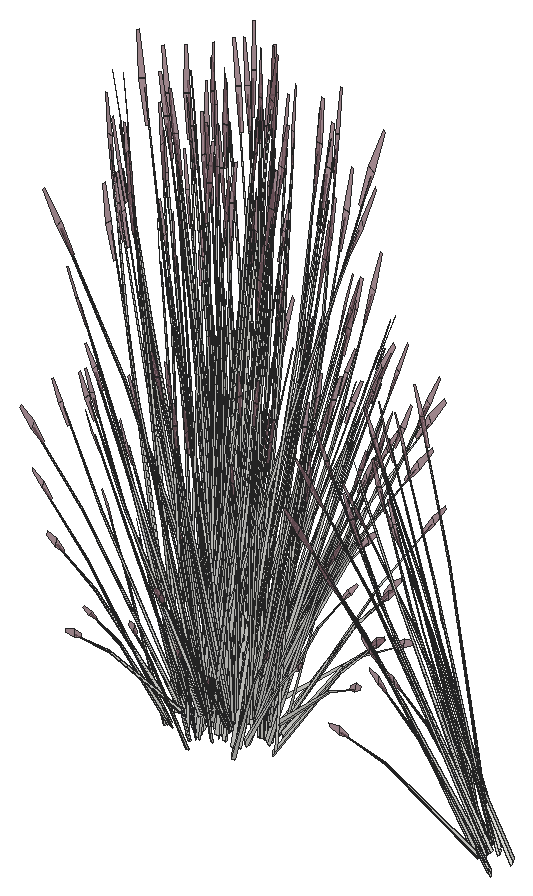
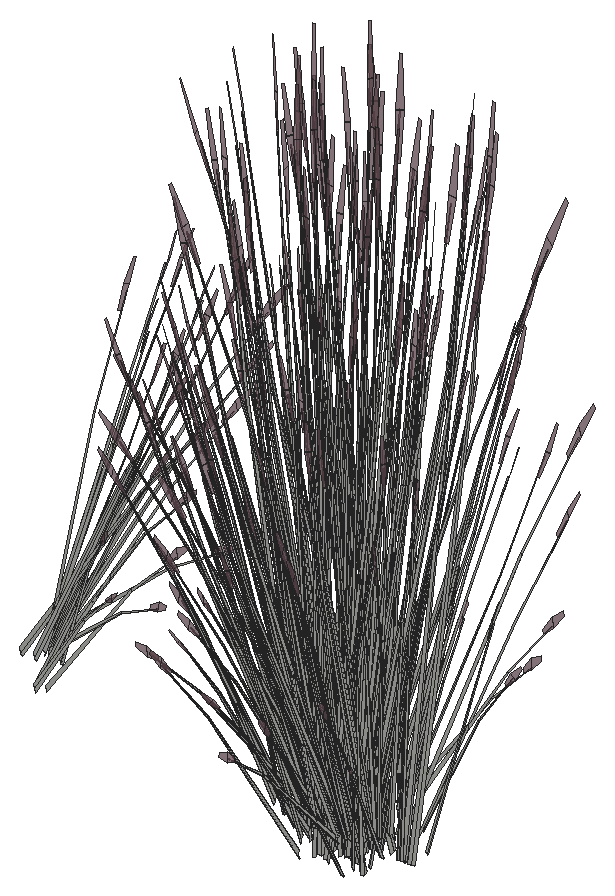
# SketchUp Ruby script. Lengths in inches.
U = 1.inch
M = Sketchup.active_model
def pt(a) = Geom::Point3d.new(a.map { |v| v * U })
def face(e, loops, mat)
  f = e.add_face(loops[0].map { |a| pt(a) })
  loops[1..].each { |l| e.add_face(l.map { |a| pt(a) }).erase! }
  f.material = f.back_material = mat if mat
  f
end
# faces: each face lists its corners as indices into pts; further lists are holes
def faces(e, pts, list, mat = nil) = list.each { |f| face(e, (f[0].is_a?(Array) ? f : [f]).map { |l| l.map { |i| pts[i] } }, mat) }
# xy, xz, yz: faces in a plane at the given z, y or x. An outline is a flat list of corners, or four numbers for a rectangle; further outlines are holes
def ring(l) = l.size == 4 ? [[l[0], l[1]], [l[2], l[1]], [l[2], l[3]], [l[0], l[3]]] : l.each_slice(2).to_a
def flat(e, list, mat, &to3) = list.each { |f| face(e, (f[0].is_a?(Array) ? f : [f]).map { |l| ring(l).map { |u, v| to3.(u, v) } }, mat) }
def xy(e, z, list, mat = nil) = flat(e, list, mat) { |x, y| [x, y, z] }
def xz(e, y, list, mat = nil) = flat(e, list, mat) { |x, z| [x, y, z] }
def yz(e, x, list, mat = nil) = flat(e, list, mat) { |y, z| [x, y, z] }
def lines(e, pts, list) = list.each { |a, b| e.add_line(pt(pts[a]), pt(pts[b])) }
# prism: a flat outline (further loops are holes) pulled along v
def prism(e, loops, v, mat = nil)
  f = face(e, loops, mat); d = Geom::Vector3d.new(v.map { |x| x * U })
  f.pushpull(f.normal.samedirection?(d) ? d.length : -d.length)
end
def box(e, o, s, mat = nil) = prism(e, [[o, [o[0] + s[0], o[1], o[2]], [o[0] + s[0], o[1] + s[1], o[2]], [o[0], o[1] + s[1], o[2]]]], [0, 0, s[2]], mat)
def at(x, y, z, deg = 0) = Geom::Transformation.translation(pt([x, y, z])) * Geom::Transformation.rotation(ORIGIN, Z_AXIS, deg.degrees)
def axes(o, x, y, z) = Geom::Transformation.new([*x, 0, *y, 0, *z, 0, *pt(o).to_a, 1])
def part(name) = M.definitions.add(name)
# library, detail: a bought-in or finely detailed component or shape, given as its bounding box
def library(name, o, s) = part(name).tap { |d| box(d.entities, o, s) }
def detail(e, o, s) = box(e.add_group.entities, o, s)
def put(e, d, t, mat = nil) = e.add_instance(d, t).tap { |i| i.material = mat if mat }
def group(e, t, mat = nil) = e.add_group.tap { |g| g.transformation = t; g.material = mat if mat }.entities
root = M.entities
M.materials.add("LightPink_Translucent").color = [144, 107, 117]
M.materials["LightPink_Translucent"].alpha = 0.75
c1 = part("blade")
p = [[2.15,0.21,22],[0,0.17,0],[0.09,0.45,0],[2.18,0.31,22],[2.29,0.31,22],[0.38,0.45,0],
  [2.48,0.24,33],[2.49,0.24,33],[2.48,0.22,33]]
faces(c1.entities,p,[[0,1,2,3],[4,5,2,3],[6,3,4,7],[8,0,3,6]])
c2 = part("seeds")
p = [[0.3,-0.1,1.38],[-0.01,-0.03,1.59],[-0.01,-0.03,0.03],[0.14,-0.07,-0.07],[0.29,-0.03,3],[0.15,0.01,3.11]]
faces(c2.entities,p,[[0,1,2,3],[1,0,4,5]],"LightPink_Translucent")
c3 = part("blade with seeds")
put(c3.entities,c1,at(0,0,0))
put(c3.entities,c2,axes([2.4,0.25,30.99],[1.5799,-0.05474,1.17369],[-0.12525,1.92788,0.29478],[-0.07173,-0.02425,1.56792]))
put(root,c3,axes([821.01,272.59,2.53],[0.40003,-0.04673,0.17707],[0.10563,0.26712,-0.2286],[-0.11464,0.07175,0.4374]))
put(root,c3,axes([821.24,273.87,1.3],[0.14502,-0.05158,0.71501],[0.35805,0.15552,-0.15377],[-0.10657,0.13457,0.3057]))
put(root,c3,axes([821.03,270.93,1.0625],[-0.13257,0.26698,-0.01946],[-0.40802,-0.08212,-0.08825],[-0.06195,-0.04367,0.29107]))
put(root,c3,axes([822.09,270.02,2.35],[-0.00857,0.03919,0.88692],[-0.42284,0.14223,-0.08381],[-0.12443,-0.0727,0.15695]))
put(root,c3,axes([821.64,270.59,1.3],[-0.02783,0.10696,0.71501],[-0.40683,0.08954,-0.15377],[-0.0951,-0.13825,0.3057]))
put(root,c3,axes([821.77,270.87,1.9375],[0.10505,0.10498,0.85688],[-0.48542,0.08838,0.06928],[-0.10971,-0.1648,0.36631]))
put(root,c3,axes([822.67,272.62,1.33],[-0.46399,0.21707,-0.14548],[-0.30855,-0.30672,-0.25001],[-0.11448,-0.03115,0.79854]))
put(root,c3,axes([821.38,273.3,2.37],[-0.32725,-0.22308,0.24001],[0.34753,-0.1924,0.1979],[-0.06036,0.10466,0.49665]))
put(root,c3,axes([821.94,270.8125,2.26],[-0.07098,-0.26335,-0.17707],[0.40574,-0.06954,0.2286],[-0.10898,-0.07547,0.4374]))
put(root,c3,axes([820.81,272.14,1.1875],[-0.57465,0,0],[0,-0.36542,-0.25804],[0,-0.08323,0.81856]))
put(root,c3,axes([821.62,273.07,1.01],[-0.10795,-0.28489,-0.15489],[0.42874,-0.0809,0.15489],[-0.08643,-0.03285,0.69487]))
put(root,c3,axes([821.26,273.28,2.37],[-0.37765,-0.01523,0.03215],[0.01035,-0.23004,0.2531],[-0.03952,0.08812,0.38595]))
put(root,c3,axes([821.38,273.37,2.26],[-0.31095,0.17214,-0.17707],[-0.29435,-0.19656,0.2286],[-0.04479,0.09987,0.4374]))
put(root,c3,axes([822.98,272.86,1.03],[-0.30954,0.24575,-0.31177],[-0.38452,-0.22284,-0.08182],[-0.12404,0.0613,0.68817]))
put(root,c3,axes([822.18,271.03,2.53],[0.07098,0.26335,0.17707],[-0.40574,0.06954,-0.2286],[-0.10898,-0.07547,0.4374]))
put(root,c3,axes([820.28,273.98,2.35],[0.05214,-0.01974,0.88692],[0.43092,0.1313,-0.08381],[-0.01013,0.10932,0.15695]))
put(root,c3,axes([821.26,272.05,1.17],[-0.42746,0.27488,0.15378],[-0.42772,-0.27199,-0.18246],[-0.01493,-0.07806,0.82443]))
put(root,c3,axes([823.01,272.81,1.66],[0.39713,0.13184,0.7563],[-0.38905,0.28403,0.29908],[-0.17427,-0.16834,0.63403]))
put(root,c3,axes([821.5,270.42,1.38],[0.23972,0.1138,0.5743],[-0.34912,0.06841,0.42196],[-0.0747,-0.08746,0.12649]))
put(root,c3,axes([823.1875,272.72,1.23],[-0.44875,-0.26316,-0.12596],[0.3776,-0.2955,0.27565],[-0.12084,0.03078,0.84108]))
put(root,c3,axes([822.37,272.46,1.11],[-0.27607,-0.27443,-0.2237],[0.41817,-0.19325,0.10766],[-0.08934,-0.03396,0.71822]))
put(root,c3,axes([821.59,273.1875,2.67],[-0.01196,0.30243,-0.3943],[-0.50354,-0.02031,0.04758],[-0.05314,0.12813,0.55778]))
put(root,c3,axes([821.58,274.04,1.38],[-0.01189,-0.19441,0.5743],[0.29719,0.13866,0.42196],[-0.05845,0.09266,0.12649]))
put(root,c3,axes([822,270.72,2.55],[0.51193,-0.08404,0.26881],[0.08885,0.32966,0.22165],[-0.1204,-0.09716,0.55625]))
put(root,c3,axes([822.96,272.66,1.11],[-0.49904,0.02018,-0.2237],[-0.04513,-0.33504,0.10766],[-0.08934,0.03396,0.71822]))
put(root,c3,axes([822.12,270.79,2.37],[0.20887,-0.2077,0.03215],[0.29744,0.12092,0.2531],[-0.09616,-0.06659,0.38595]))
put(root,c3,axes([822.01,273.22,1.24],[0.4301,0.16348,0.24825],[-0.25708,0.29314,0],[-0.09796,-0.03723,0.78752]))
put(root,c3,axes([821.42,273.61,1.68],[0.0101,-0.16879,0.77173],[0.45413,0.08915,0.10664],[-0.03935,0.17989,0.36441]))
put(root,c3,axes([822.41,272.62,1.22],[0.1218,-0.38743,-0.11714],[0.57753,0.06753,0.25635],[-0.10091,-0.0535,0.7822]))
put(root,c3,axes([822.62,272.71,1.31],[-0.08866,0.29179,0.0724],[-0.43315,-0.05065,-0.20674],[-0.07883,-0.02996,0.63372]))
put(root,c3,axes([822.57,270.17,2.36],[-0.07029,-0.04584,0.87472],[-0.46908,0.02906,-0.13834],[-0.07486,-0.10965,0.07015]))
put(root,c3,axes([823.48,273.53,1.01],[-0.4301,0.16348,-0.24825],[-0.25708,-0.29314,0],[-0.09796,0.03723,0.78752]))
put(root,c3,axes([820.9375,271.9,1.01],[0,-0.32696,-0.24825],[0.51416,0,0],[0,-0.07447,0.78752]))
put(root,c3,axes([821.16,272.2,1.24],[0,0.32696,0.24825],[-0.51416,0,0],[0,-0.07447,0.78752]))
put(root,c3,axes([823.51,273.4375,1.1],[-0.28374,-0.32877,-0.02571],[0.4807,-0.18271,0.25804],[-0.11845,0.0313,0.81815]))
put(root,c3,axes([821.69,273.29,2.5],[0.32898,0.21969,-0.2836],[-0.34753,0.1924,-0.21967],[-0.05006,0.11162,0.54264]))
put(root,c3,axes([823.38,273.4,1.01],[-0.42874,-0.0809,-0.15489],[0.10795,-0.28489,0.15489],[-0.08643,0.03285,0.69487]))
put(root,c3,axes([821.55,273.125,2.53],[0.31095,-0.17214,0.17707],[0.29435,0.19656,-0.2286],[-0.04479,0.09987,0.4374]))
put(root,c3,axes([822.28,272.28,1.33],[-0.51755,-0.15601,-0.14548],[0.2492,-0.32927,-0.25001],[-0.01626,-0.08084,0.79854]))
put(root,c3,axes([823.63,272.18,1.42],[-0.01255,-0.30784,0.70636],[0.56816,0.0798,0.29908],[-0.13438,0.16845,0.66675]))
put(root,c3,axes([821.35,273.17,2.7],[0.50507,0.0162,-0.06749],[-0.01381,0.30672,-0.3746],[-0.03508,0.11813,0.56919]))
put(root,c3,axes([821.34,273.62,1.41],[0.41748,-0.0579,0.03254],[0.09598,0.23326,-0.43152],[-0.02647,0.11808,0.3868]))
put(root,c3,axes([823.3125,272.57,1.33],[0.05355,0.37308,-0.14548],[-0.55775,0.02256,-0.25001],[-0.09822,0.04969,0.79854]))
put(root,c3,axes([822.05,271.94,1.05],[-0.18873,-0.33528,-0.34918],[0.54365,-0.12075,-0.09164],[-0.02086,-0.11353,0.77075]))
put(root,c3,axes([823.29,270.88,2.52],[-0.44971,0.15222,-0.0608],[-0.221,-0.27017,-0.33747],[-0.05933,-0.11385,0.51278]))
put(root,c3,axes([822.9,270.89,2.34],[-0.45175,-0.08196,-0.25549],[0.15485,-0.28101,-0.1979],[-0.04142,-0.11314,0.48886]))
put(root,c3,axes([822.07,272.97,1.9375],[-0.01125,-0.12549,0.85688],[0.48751,0.08325,0.06928],[-0.03015,0.17883,0.36631]))
put(root,c3,axes([821.16,271.9,1.01],[0.32079,-0.20399,-0.15489],[0.32079,0.20399,0.15489],[0,-0.06571,0.69487]))
put(root,c3,axes([822.61,270.58,1.0625],[-0.31757,0.18757,-0.01946],[-0.29098,-0.20543,-0.08825],[-0.02049,-0.05821,0.29107]))
put(root,c3,axes([822.48,272.43,1.18],[0.58084,0.06889,0.22877],[-0.11821,0.38906,0.08977],[-0.08488,-0.03757,0.79428]))
put(root,c3,axes([822.33,272.36,1.36],[-0.22297,0.29461,0.2237],[-0.4633,-0.14179,-0.10766],[0,-0.06791,0.71822]))
put(root,c3,axes([823.07,270.95,2.49],[-0.21934,-0.26585,-0.35523],[0.45151,-0.14816,0.04287],[-0.05129,-0.12845,0.5025]))
put(root,c3,axes([822.17,273.06,1.24],[0.49383,-0.08678,0.08821],[0.12194,0.32295,0.17543],[-0.04404,-0.04705,0.80203]))
put(root,c3,axes([822.8,273.11,1.1],[-0.4633,-0.14679,0],[0.22297,-0.30501,0],[0,0,0.81353]))
put(root,c3,axes([823.15,270.98,2.53],[-0.13855,0.25143,0.17707],[-0.4042,-0.07334,-0.2286],[-0.03706,-0.10123,0.4374]))
put(root,c3,axes([823.875,273.48,1.1875],[0.28732,0.32763,0],[-0.4807,0.18271,-0.25804],[-0.10948,0.04161,0.81856]))
put(root,c3,axes([822.41,273.62,2.53],[-0.45283,-0.08548,0.26641],[0.15485,-0.28101,0.21967],[0.02721,0.11051,0.55128]))
put(root,c3,axes([822.29,273.64,2.37],[-0.33863,0.11112,0.03215],[-0.16575,-0.20263,0.2531],[0.0327,0.08932,0.38595]))
put(root,c3,axes([823.64,273.07,1.24],[0.13276,-0.32494,0.08821],[0.4858,0.09195,0.17543],[-0.08392,0.00158,0.80203]))
put(root,c3,axes([823.41,272.64,1.31],[0.33952,0.19644,0.0724],[-0.2832,0.22163,-0.20674],[-0.07883,0.02996,0.63372]))
put(root,c3,axes([823.29,272.4,1.15],[-0.42746,-0.28142,-0.03066],[0.42772,-0.28159,0],[-0.01493,-0.00983,0.87786]))
put(root,c3,axes([823.4,272.5,1.36],[0.49904,-0.02018,0.2237],[0.04513,0.33504,-0.10766],[-0.08934,0.03396,0.71822]))
put(root,c3,axes([823.53,273.27,1.17],[0.57533,0.10627,0.15378],[-0.14394,0.37986,-0.18246],[-0.09522,0.04754,0.82443]))
put(root,c3,axes([822.6875,270.36,0.75],[-0.07708,0.01178,0.88171],[-0.42627,-0.1326,-0.1347],[0.00715,-0.1106,0.15018]))
put(root,c3,axes([823.77,273.25,1.24],[0.4301,-0.16348,0.24825],[0.25708,0.29314,0],[-0.09796,0.03723,0.78752]))
put(root,c3,axes([823.11,270.72,2.26],[0.13855,-0.25143,-0.17707],[0.4042,0.07334,0.2286],[-0.03706,-0.10123,0.4374]))
put(root,c3,axes([822.43,272.08,1.18],[0.1998,0.3656,0.22877],[-0.5709,0.12713,0.08977],[0.00698,-0.06718,0.79428]))
put(root,c3,axes([822.34,272.03,1.11],[0.22297,-0.29461,-0.2237],[0.4633,0.14179,0.10766],[0,-0.06791,0.71822]))
put(root,c3,axes([822.91,272.98,1.1],[-0.14994,-0.28188,0],[0.42817,-0.09871,0],[0,0,0.77185]))
put(root,c3,axes([822.36,273.57,0.75],[0.07437,-0.01779,0.88171],[0.44738,0.09793,-0.1347],[0.01308,0.11037,0.15018]))
put(root,c3,axes([822.46,273.67,2.26],[-0.13855,0.25143,-0.17707],[-0.4042,-0.07334,0.2286],[0.03706,0.10123,0.4374]))
put(root,c3,axes([823.51,272.42,1.11],[-0.22297,0.29461,-0.2237],[-0.4633,-0.14179,0.10766],[0,0.06791,0.71822]))
put(root,c3,axes([823.28,270.76,2.37],[0.33863,-0.11112,0.03215],[0.16575,0.20263,0.2531],[-0.0327,-0.08932,0.38595]))
put(root,c3,axes([822.18,274.12,2.36],[0.05825,0.05265,0.87472],[0.47011,0.02068,-0.13834],[0.04727,0.11612,0.07015]))
put(root,c3,axes([824.4,272.25,1.24],[-0.36107,-0.23816,0.08821],[0.36387,-0.231,0.17543],[-0.03988,0.04864,0.80203]))
put(root,c3,axes([823.15,272.11,1.1],[0,-0.37831,0],[0.57465,0,0],[0,0,0.89728]))
put(root,c3,axes([823.16,270.78,2.37],[0.45283,0.08548,0.24001],[-0.15485,0.28101,0.1979],[-0.02721,-0.11051,0.49665]))
put(root,c3,axes([822.61,272.18,1.22],[0.5178,0.15847,0.12032],[-0.2492,0.32927,0.25001],[0,-0.0759,0.80271]))
put(root,c3,axes([823.4375,272.26,1.15],[0,0.37813,-0.02818],[-0.57465,0,0],[0,0.01188,0.89684]))
put(root,c3,axes([822.45,271.96,1.36],[-0.49904,0.02018,0.2237],[-0.04513,-0.33504,-0.10766],[0.08934,-0.03396,0.71822]))
put(root,c3,axes([822.42,273.41,2.53],[0.13855,-0.25143,0.17707],[0.4042,0.07334,-0.2286],[0.03706,0.10123,0.4374]))
put(root,c3,axes([822.21,271.38,1.24],[-0.13276,0.32494,0.08821],[-0.4858,-0.09195,0.17543],[0.08392,-0.00158,0.80203]))
put(root,c3,axes([823.16,272.99,1.15],[0.1998,0.37562,-0.03006],[-0.5709,0.13162,0],[0.00698,0.01312,0.86086]))
put(root,c3,axes([821.98,270.98,1.1875],[-0.28732,-0.32763,0],[0.4807,-0.18271,-0.25804],[0.10948,-0.04161,0.81856]))
put(root,c3,axes([822.5,273.45,2.49],[0.21934,0.26585,-0.35523],[-0.45151,0.14816,0.04287],[0.05129,0.12845,0.5025]))
put(root,c3,axes([824.8125,272.5,1.1],[-0.57436,-0.00261,-0.02488],[0,-0.36542,0.24971],[-0.01805,0.08319,0.79176]))
put(root,c3,axes([823.68,271.4,1.24],[-0.49383,0.08678,0.08821],[-0.12194,-0.32295,0.17543],[0.04404,0.04705,0.80203]))
put(root,c3,axes([823.18,270.1875,1.38],[0.05895,0.19066,0.5743],[-0.32704,-0.1056,0.42196],[0.03519,-0.09762,0.12649]))
put(root,c3,axes([822.96,274.31,2.82],[0.31757,-0.18757,-0.03244],[0.29098,0.20543,-0.14708],[0.02049,0.05821,0.48512]))
put(root,c3,axes([822.875,271.87,1.18],[-0.38104,0.29672,0.22877],[-0.45269,-0.26192,0.08977],[0.09186,-0.02961,0.79428]))
put(root,c3,axes([823.53,272.34,1.11],[0.32079,0.21119,0],[-0.32079,0.21119,0],[0,0,0.84633]))
put(root,c3,axes([823.52,272.09,1.36],[0.22297,-0.29461,0.2237],[0.4633,0.14179,-0.10766],[0,0.06791,0.71822]))
put(root,c3,axes([823.33,273.11,1.1],[0.4633,0.14679,0],[-0.22297,0.30501,0],[0,0,0.87477]))
put(root,c3,axes([822.67,273.5,2.34],[0.45175,0.08196,-0.25549],[-0.15485,0.28101,-0.1979],[0.04142,0.11314,0.48886]))
put(root,c3,axes([822.28,273.52,2.52],[0.44971,-0.15222,-0.0608],[0.221,0.27017,-0.33747],[0.05933,0.11385,0.51278]))
put(root,c3,axes([823.37,272.02,1.19],[-0.58084,-0.06889,0.24599],[0.11821,-0.38906,0.09653],[0.08488,0.03757,0.85407]))
put(root,c3,axes([824.58,270.5,2.35],[-0.04667,0.02497,0.88692],[-0.45726,-0.08426,-0.08381],[-0.01655,-0.10898,0.15695]))
put(root,c3,axes([824.22,271.22,2.52],[-0.50507,-0.0162,-0.0608],[0.01381,-0.30672,-0.33747],[0.03508,-0.11813,0.51278]))
put(root,c3,axes([824.69,272.55,1.01],[-0.32079,0.20399,-0.15489],[-0.32079,-0.20399,0.15489],[0,0.06571,0.69487]))
put(root,c3,axes([823.78,272.51,1.05],[0.16851,0.29936,-0.34606],[-0.4854,0.10781,-0.09083],[0.01863,0.10137,0.76386]))
put(root,c3,axes([823.54,272.19,1.1],[0.51416,0,0],[0,0.33849,0],[0,0,0.89203]))
put(root,c3,axes([824.02,271.27,2.53],[-0.31095,0.17214,0.17707],[-0.29435,-0.19656,-0.2286],[0.04479,-0.09987,0.4374]))
put(root,c3,axes([823.04,271.82,1.36],[-0.27607,-0.27443,0.2237],[0.41817,-0.19325,-0.10766],[0.08934,0.03396,0.71822]))
put(root,c3,axes([822.54,271.88,1.33],[-0.05355,-0.37308,-0.14548],[0.55775,-0.02256,-0.25001],[0.09822,-0.04969,0.79854]))
put(root,c3,axes([823.72,272.16,1.31],[0.42817,-0.09535,0.0724],[0.14994,0.27228,-0.20674],[0,0.05992,0.63372]))
put(root,c3,axes([823.875,271.1,2.34],[-0.32898,-0.21969,-0.25549],[0.34753,-0.1924,-0.1979],[0.05006,-0.11162,0.48886]))
put(root,c3,axes([823.57,272.18,1.33],[0.51755,0.15601,-0.14548],[-0.2492,0.32927,-0.25001],[0.01626,0.08084,0.79854]))
put(root,c3,axes([822.47,271.06,1.01],[0.42874,0.0809,-0.15489],[-0.10795,0.28489,0.15489],[0.08643,-0.03285,0.69487]))
put(root,c3,axes([823.66,270.71,1.3],[-0.13063,0.06618,0.71501],[-0.39122,-0.11583,-0.15377],[0.07252,-0.14406,0.3057]))
put(root,c3,axes([824.69,272.25,1.24],[0,-0.32696,0.24825],[0.51416,0,0],[0,0.07447,0.78752]))
put(root,c3,axes([824.91,272.56,1.01],[0,0.32696,-0.24825],[-0.51416,0,0],[0,0.07447,0.78752]))
put(root,c3,axes([823.54,273.55,2.37],[-0.45708,0.07503,0.24001],[-0.07933,-0.29434,0.1979],[0.1075,0.08675,0.49665]))
put(root,c3,axes([822.37,270.93,1.01],[0.4301,-0.16348,-0.24825],[0.25708,0.29314,0],[0.09796,-0.03723,0.78752]))
put(root,c3,axes([823.45,273.61,2.37],[-0.20887,0.2077,0.03215],[-0.29744,-0.12092,0.2531],[0.09616,0.06659,0.38595]))
put(root,c3,axes([822.93,272.92,1.9375],[-0.10505,-0.10498,0.85688],[0.48542,-0.08838,0.06928],[0.10971,0.1648,0.36631]))
put(root,c3,axes([823.23,271.74,1.31],[0.08866,-0.29179,0.0724],[0.43315,0.05065,-0.20674],[0.07883,0.02996,0.63372]))
put(root,c3,axes([823.85,271.23,1.24],[-0.4301,-0.16348,0.24825],[0.25708,-0.29314,0],[0.09796,0.03723,0.78752]))
put(root,c3,axes([823.98,271.21,2.49],[0.01196,-0.30243,-0.35523],[0.50354,0.02031,0.04287],[0.05314,-0.12813,0.5025]))
put(root,c3,axes([823.47,272.94,1.09],[0.48247,-0.11094,-0.09599],[0.16954,0.31956,0.00004],[0.05326,-0.01226,0.86949]))
put(root,c3,axes([823.39,273.37,2.53],[-0.07098,-0.26335,0.17707],[0.40574,-0.06954,-0.2286],[0.10898,0.07547,0.4374]))
put(root,c3,axes([823.48,271.99,1.11],[0.27607,0.27443,-0.2237],[-0.41817,0.19325,0.10766],[0.08934,0.03396,0.71822]))
put(root,c3,axes([823.66,271.85,2.24],[-0.39711,-0.16988,0.69141],[0.41931,-0.2645,0.29833],[0.12812,0.1594,0.66832]))
put(root,c3,axes([824.1875,271.02,2.26],[0.31095,-0.17214,-0.17707],[0.29435,0.19656,0.2286],[0.04479,-0.09987,0.4374]))
put(root,c3,axes([822.99,273.74,2.35],[0.00136,-0.03958,0.88692],[0.39383,-0.17464,-0.08381],[0.1368,0.06234,0.15695]))
put(root,c3,axes([824.31,271.11,2.37],[0.37765,0.01523,0.03215],[-0.01035,0.23004,0.2531],[0.03952,-0.08812,0.38595]))
put(root,c3,axes([824.26,273.24,1.38],[-0.25875,-0.09401,0.5743],[0.33411,-0.09552,0.42196],[0.09012,0.08091,0.12649]))
put(root,c3,axes([823.34,273.14,1.3],[0.00811,-0.10838,0.71501],[0.38755,-0.12106,-0.15377],[0.11964,0.12972,0.3057]))
put(root,c3,axes([824.68,270.73,2.36],[-0.00444,-0.06507,0.87472],[-0.37468,-0.18807,-0.13834],[0.05793,-0.114,0.07015]))
put(root,c3,axes([822.875,271.6,1.03],[0.30954,-0.24575,-0.31177],[0.38452,0.22284,-0.08182],[0.12404,-0.0613,0.68817]))
put(root,c3,axes([824.19,271.09,2.37],[0.32725,0.22308,0.24001],[-0.34753,0.1924,0.1979],[0.06036,-0.10466,0.49665]))
put(root,c3,axes([824.23,271.38,1.01],[0.10795,0.28489,-0.15489],[-0.42874,0.0809,0.15489],[0.08643,0.03285,0.69487]))
put(root,c3,axes([825.04,272.31,1.1875],[0.57465,0,0],[0,0.36542,-0.25804],[0,0.08323,0.81856]))
put(root,c3,axes([823.19,271.84,1.33],[0.46399,-0.21707,-0.14548],[0.30855,0.30672,-0.25001],[0.11448,0.03115,0.79854]))
put(root,c3,axes([824.3,273.66,1.33],[-0.2947,-0.01025,0.5253],[0.19462,-0.21779,0.29003],[0.11642,0.07737,0.41205]))
put(root,c3,axes([824.5625,271.8,2.53],[-0.40003,0.04673,0.17707],[-0.10563,-0.26712,-0.2286],[0.11464,-0.07175,0.4374]))
put(root,c3,axes([823.41,271.05,1.9375],[-0.08557,0.11238,0.85688],[-0.35897,-0.23257,0.06928],[0.16194,-0.14495,0.36631]))
put(root,c3,axes([823.35,273.5,2.52],[0.27385,-0.27986,-0.0608],[0.39658,0.16123,-0.33747],[0.13785,0.07907,0.51278]))
put(root,c3,axes([822.01,271.64,0.8],[-0.45234,0.1309,0.64464],[-0.14398,-0.37559,0.25048],[0.27777,0.00625,0.73321]))
put(root,c3,axes([824.77,271.82,2.52],[-0.4251,-0.18028,-0.0608],[0.24491,-0.26108,-0.33747],[0.1201,-0.09075,0.51278]))
put(root,c3,axes([823.68,273.37,2.34],[0.45348,-0.07772,-0.25549],[0.07933,0.29434,-0.1979],[0.1218,0.08435,0.48886]))
put(root,c3,axes([824.09,271.0625,1.1875],[0.28732,-0.32763,0],[0.4807,0.18271,-0.25804],[0.10948,0.04161,0.81856]))
put(root,c3,axes([824.57,270.92,0.75],[-0.06878,-0.02576,0.88171],[-0.17668,-0.28776,-0.1347],[0.11919,-0.07809,0.15018]))
put(root,c3,axes([824.2,273.01,2.53],[-0.26148,-0.20471,0.17707],[0.29857,-0.19378,-0.2286],[0.1517,0.02948,0.4374]))
put(root,c3,axes([824.35,271.26,1.01],[0.4301,0.16348,-0.24825],[-0.25708,0.29314,0],[0.09796,0.03723,0.78752]))
put(root,c3,axes([824.43,273.2,2.37],[-0.02314,0.24862,0.03215],[-0.34943,-0.00682,0.2531],[0.13385,0.02602,0.38595]))
put(root,c3,axes([824.33,273.59,0.75],[0.03348,-0.0472,0.88171],[0.42153,-0.13902,-0.1347],[0.12779,0.07195,0.15018]))
put(root,c3,axes([824.47,273.12,2.37],[-0.33886,0.21544,0.24001],[-0.29224,-0.22879,0.1979],[0.15898,0.03974,0.49665]))
put(root,c3,axes([824.56,271.61,2.34],[-0.11806,-0.29854,-0.25549],[0.44709,-0.05222,-0.1979],[0.12812,-0.08019,0.48886]))
put(root,c3,axes([825.35,273.15,1.96],[-0.08796,-0.27485,-0.01746],[0.41573,-0.06319,-0.07916],[0.08682,0.01742,0.26109]))
put(root,c3,axes([824.63,272.4375,2.53],[-0.38192,-0.09121,0.17707],[0.11139,-0.2661,-0.2286],[0.15377,-0.0244,0.4374]))
put(root,c3,axes([823.73,271.89,1.03],[0.47805,0.0536,-0.31177],[-0.10088,0.33065,-0.08182],[0.14266,0.04007,0.68817]))
put(root,c3,axes([825.76,272.08,1.13],[-0.28491,-0.20907,-0.03244],[0.31204,-0.19157,-0.14708],[0.08842,-0.01349,0.48512]))
put(root,c3,axes([825.11,271.02,1.38],[-0.15307,0.16644,0.5743],[-0.13157,-0.22361,0.42196],[0.12643,-0.05603,0.12649]))
put(root,c3,axes([824.93,271.76,2.37],[0.31549,0.13751,0.03215],[-0.18368,0.19581,0.2531],[0.10115,-0.06331,0.38595]))
put(root,c3,axes([824.84,271.7,2.37],[0.11397,0.30091,0.24001],[-0.44709,0.05222,0.1979],[0.13177,-0.07077,0.49665]))
put(root,c3,axes([823.63,272.59,1.9375],[-0.1707,-0.05633,0.85688],[0.35326,-0.23632,0.06928],[0.22018,0.10661,0.36631]))
put(root,c3,axes([825.82,271.75,2.35],[-0.06002,-0.00248,0.88692],[-0.24926,-0.26607,-0.08381],[0.1001,-0.08748,0.15695]))
put(root,c3,axes([824.89,271.64,2.26],[0.40003,-0.04673,-0.17707],[0.10563,0.26712,0.2286],[0.11464,-0.07175,0.4374]))
put(root,c3,axes([824.57,271.73,2.49],[0.24005,-0.25798,-0.35523],[0.42065,0.18334,0.04287],[0.14333,-0.09347,0.5025]))
put(root,c3,axes([824.97,272.52,2.37],[0.16879,0.22293,0.03215],[-0.30779,0.10912,0.2531],[0.13568,-0.02153,0.38595]))
put(root,c3,axes([824.57,273.12,2.26],[0.26148,0.20471,-0.17707],[-0.29857,0.19378,0.2286],[0.1517,0.02948,0.4374]))
put(root,c3,axes([824.27,273.14,2.52],[0.02461,-0.33251,-0.0608],[0.4659,0.00909,-0.33747],[0.17944,0.0231,0.51278]))
put(root,c3,axes([824.79,272.53,2.52],[-0.23123,-0.29606,-0.0608],[0.41039,-0.14549,-0.33747],[0.17294,-0.03906,0.51278]))
put(root,c3,axes([824.94,272.44,2.37],[-0.12984,0.29812,0.24001],[-0.42685,-0.10194,0.1979],[0.16786,-0.01792,0.49665]))
put(root,c3,axes([824.67,272.94,2.36],[0.09858,-0.00553,0.87472],[0.2704,-0.25401,-0.13834],[0.17535,0.03353,0.07015]))
put(root,c3,axes([824.77,272.27,2.34],[0.1245,-0.29741,-0.25549],[0.42685,0.10194,-0.1979],[0.17186,-0.02727,0.48886]))
put(root,c3,axes([825.84,272.46,1.38],[-0.28394,0.05398,0.5743],[0.13365,-0.22308,0.42196],[0.15063,0.01526,0.12649]))
put(root,c3,axes([824.92,271.49,1.3],[-0.16417,-0.00968,0.71501],[-0.16819,-0.25979,-0.15377],[0.20169,-0.07349,0.3057]))
put(root,c3,axes([825.03,272.41,2.26],[0.38192,0.09121,-0.17707],[-0.11139,0.2661,0.2286],[0.15377,-0.0244,0.4374]))
put(root,c3,axes([824.29,272.98,2.49],[0.45939,0.00787,-0.35523],[-0.03085,0.3315,0.04287],[0.19462,0.03498,0.5025]))
put(root,c3,axes([825.22,272.36,0.99],[-0.29599,0.03924,0.70792],[-0.04711,-0.31232,0.04052],[0.20731,-0.04727,0.40283]))
put(root,c3,axes([825.55,272.15,0.75],[-0.02402,-0.04964,0.88171],[0.16658,-0.29036,-0.1347],[0.16804,-0.00418,0.15018]))
put(root,c3,axes([825.71,273.41,2.35],[-0.04155,-0.02862,0.88692],[0.0909,-0.30682,-0.08381],[0.16368,-0.0196,0.15695]))
put(root,c3,axes([823.99,272.08,1.9375],[-0.19062,0.00741,0.85688],[0.12645,-0.32094,0.06928],[0.27165,0.01985,0.36631]))
put(root,c3,axes([824.6875,272.38,2.49],[0.40382,-0.1444,-0.35523],[0.22505,0.29724,0.04287],[0.19512,-0.03377,0.5025]))
put(root,c3,axes([826.04,272.0625,2.36],[0.06377,-0.0498,0.87472],[-0.08162,-0.30549,-0.13834],[0.16001,-0.05792,0.07015]))
put(root,c3,axes([825.31,272.82,1.3],[-0.11068,-0.08041,0.71501],[0.144,-0.26601,-0.15377],[0.22393,0.03604,0.3057]))
put(root,c3,axes([838.82,269.4,1.9375],[0.19062,-0.00741,0.85688],[-0.12645,0.32094,0.06928],[-0.27165,-0.01985,0.36631]))
put(root,c3,axes([838.9,269.96,1.9375],[0.15946,-0.06916,0.85688],[0.13424,0.31957,0.06928],[-0.25033,0.07223,0.36631]))
put(root,c3,axes([838.41,270.51,1.3],[0.15971,0.02684,0.71501],[0.10294,0.27415,-0.15377],[-0.21694,0.05132,0.3057]))
put(root,c3,axes([839.82,269.63,1.67],[0.13063,-0.0473,0.88532],[0.04505,0.33024,0.06928],[-0.28294,0.04382,0.31642]))
put(root,c3,axes([838.42,269.85,2.36],[-0.07505,0.04245,0.87472],[0.00638,0.31015,-0.13834],[-0.17202,0.04033,0.07015]))
put(root,c3,axes([839.4,269.1,2.49],[-0.45939,-0.00787,-0.35523],[0.03085,-0.3315,0.04287],[-0.19462,-0.03498,0.5025]))
put(root,c3,axes([839.02,269.18,1.3],[0.08973,0.09103,0.71501],[-0.20675,0.24743,-0.15377],[-0.2123,-0.05914,0.3057]))
put(root,c3,axes([838.66,269.67,2.26],[-0.38192,-0.09121,-0.17707],[0.11139,-0.2661,0.2286],[-0.15377,0.0244,0.4374]))
put(root,c3,axes([839.19,268.88,1.9375],[0.1707,0.05633,0.85688],[-0.35326,0.23632,0.06928],[-0.22018,-0.10661,0.36631]))
put(root,c3,axes([837.58,270.17,2.35],[0.05865,0.00877,0.88692],[0.18143,0.28888,-0.08381],[-0.12006,0.07582,0.15695]))
put(root,c3,axes([838.92,269.81,2.34],[-0.1245,0.29741,-0.25549],[-0.42685,-0.10194,-0.1979],[-0.17186,0.02727,0.48886]))
put(root,c3,axes([839.24,269.17,2.34],[-0.3337,0.21658,-0.25549],[-0.29224,-0.22879,-0.1979],[-0.16955,-0.03295,0.48886]))
put(root,c3,axes([838.7,269.79,0.75],[0.01165,0.05153,0.88171],[-0.23495,0.26909,-0.1347],[-0.16689,-0.01356,0.15018]))
put(root,c3,axes([838.77,268.5625,2.35],[0.03407,0.03263,0.88692],[-0.16424,0.29331,-0.08381],[-0.16634,0.00212,0.15695]))
put(root,c3,axes([838.07,271.08,1.38],[0.19152,-0.14818,0.5743],[0.07557,0.23459,0.42196],[-0.13841,0.042,0.12649]))
put(root,c3,axes([839.15,268.37,2.36],[-0.09888,-0.00231,0.87472],[-0.3148,0.23079,-0.13834],[-0.16797,-0.04716,0.07015]))
put(root,c3,axes([838.75,269.64,2.37],[0.12984,-0.29812,0.24001],[0.42685,0.10194,0.1979],[-0.16786,0.01792,0.49665]))
put(root,c3,axes([838.9,269.56,2.52],[0.23123,0.29606,-0.0608],[-0.41039,0.14549,-0.33747],[-0.17294,0.03906,0.51278]))
put(root,c3,axes([839.42,268.94,2.52],[-0.02461,0.33251,-0.0608],[-0.4659,-0.00909,-0.33747],[-0.17944,-0.0231,0.51278]))
put(root,c3,axes([839.12,268.96,2.26],[-0.26148,-0.20471,-0.17707],[0.29857,-0.19378,0.2286],[-0.1517,-0.02948,0.4374]))
put(root,c3,axes([838.71,269.5625,2.37],[-0.16879,-0.22293,0.03215],[0.30779,-0.10912,0.2531],[-0.13568,0.02153,0.38595]))
